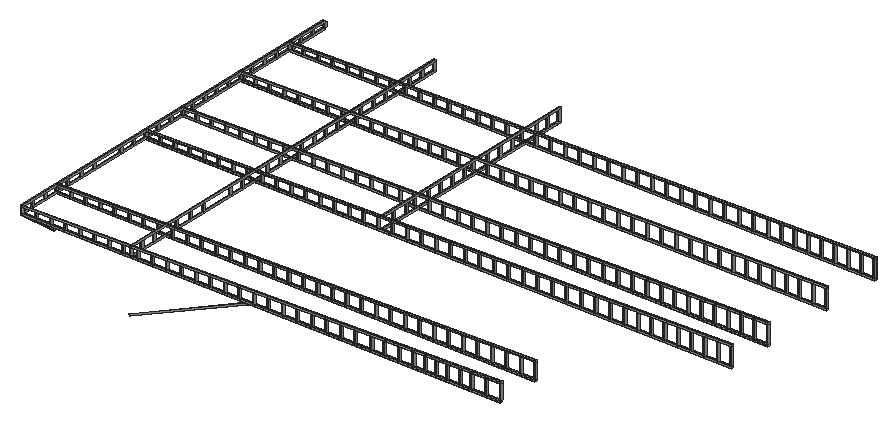
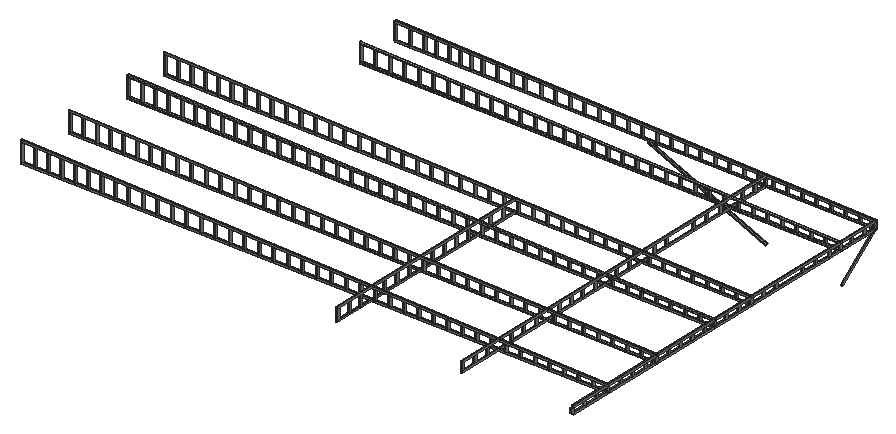
# SketchUp Ruby script. Lengths in millimetres.
U = 1.mm
M = Sketchup.active_model
def pt(a) = Geom::Point3d.new(a.map { |v| v * U })
def face(e, loops, mat)
  f = e.add_face(loops[0].map { |a| pt(a) })
  loops[1..].each { |l| e.add_face(l.map { |a| pt(a) }).erase! }
  f.material = f.back_material = mat if mat
  f
end
# faces: each face lists its corners as indices into pts; further lists are holes
def faces(e, pts, list, mat = nil) = list.each { |f| face(e, (f[0].is_a?(Array) ? f : [f]).map { |l| l.map { |i| pts[i] } }, mat) }
# xy, xz, yz: faces in a plane at the given z, y or x. An outline is a flat list of corners, or four numbers for a rectangle; further outlines are holes
def ring(l) = l.size == 4 ? [[l[0], l[1]], [l[2], l[1]], [l[2], l[3]], [l[0], l[3]]] : l.each_slice(2).to_a
def flat(e, list, mat, &to3) = list.each { |f| face(e, (f[0].is_a?(Array) ? f : [f]).map { |l| ring(l).map { |u, v| to3.(u, v) } }, mat) }
def xy(e, z, list, mat = nil) = flat(e, list, mat) { |x, y| [x, y, z] }
def xz(e, y, list, mat = nil) = flat(e, list, mat) { |x, z| [x, y, z] }
def yz(e, x, list, mat = nil) = flat(e, list, mat) { |y, z| [x, y, z] }
def lines(e, pts, list) = list.each { |a, b| e.add_line(pt(pts[a]), pt(pts[b])) }
# prism: a flat outline (further loops are holes) pulled along v
def prism(e, loops, v, mat = nil)
  f = face(e, loops, mat); d = Geom::Vector3d.new(v.map { |x| x * U })
  f.pushpull(f.normal.samedirection?(d) ? d.length : -d.length)
end
def box(e, o, s, mat = nil) = prism(e, [[o, [o[0] + s[0], o[1], o[2]], [o[0] + s[0], o[1] + s[1], o[2]], [o[0], o[1] + s[1], o[2]]]], [0, 0, s[2]], mat)
def at(x, y, z, deg = 0) = Geom::Transformation.translation(pt([x, y, z])) * Geom::Transformation.rotation(ORIGIN, Z_AXIS, deg.degrees)
def axes(o, x, y, z) = Geom::Transformation.new([*x, 0, *y, 0, *z, 0, *pt(o).to_a, 1])
def part(name) = M.definitions.add(name)
# library, detail: a bought-in or finely detailed component or shape, given as its bounding box
def library(name, o, s) = part(name).tap { |d| box(d.entities, o, s) }
def detail(e, o, s) = box(e.add_group.entities, o, s)
def put(e, d, t, mat = nil) = e.add_instance(d, t).tap { |i| i.material = mat if mat }
def group(e, t, mat = nil) = e.add_group.tap { |g| g.transformation = t; g.material = mat if mat }.entities
root = M.entities
M.materials.add("[Metal Rough]").color = [153, 157, 160]
c1 = part("Group\#22")
g1 = group(c1.entities,at(0,0,300))
prism(g1,[[[27087.5,80,600],[0,80,0],[0,80,80],[27087.5,80,680]]],[0,-80,0])
g2 = group(c1.entities,at(27087.5,0,0),"[Metal Rough]")
prism(g2,[[[-27087.5,80,0],[-27087.5,0,0],[-27087.5,0,80],[-27087.5,80,80]],[[-27087.5,76,4],[-27087.5,76,76],[-27087.5,4,76],[-27087.5,4,4]]],[27087.5,0,0])
c2 = part("Group\#63")
prism(c2.entities,[[[6104.2,85,80],[6104.2,85,435.2],[6078.7,85,434.6],[6024.2,85,433.4],[6024.2,85,80]]],[0,80,0],"[Metal Rough]")
prism(c2.entities,[[[7442.9,85,80],[7442.9,85,464.9],[7417.4,85,464.3],[7362.9,85,463.1],[7362.9,85,80]]],[0,80,0],"[Metal Rough]")
prism(c2.entities,[[[6773.6,85,80],[6773.6,85,450],[6748.1,85,449.5],[6693.6,85,448.3],[6693.6,85,80]]],[0,80,0],"[Metal Rough]")
prism(c2.entities,[[[8112.3,85,80],[8112.3,85,479.7],[8086.8,85,479.1],[8032.3,85,477.9],[8032.3,85,80]]],[0,80,0],"[Metal Rough]")
prism(c2.entities,[[[5434.8,85,80],[5434.8,85,420.4],[5409.4,85,419.8],[5354.8,85,418.6],[5354.8,85,80]]],[0,80,0],"[Metal Rough]")
prism(c2.entities,[[[4096.1,85,80],[4096.1,85,390.7],[4070.6,85,390.2],[4016.1,85,388.9],[4016.1,85,80]]],[0,80,0],"[Metal Rough]")
prism(c2.entities,[[[1418.7,165,80],[1338.7,165,80],[1338.7,165,329.6],[1393.2,165,330.9],[1418.7,165,331.4]]],[0,-80,0],"[Metal Rough]")
prism(c2.entities,[[[3426.8,165,80],[3346.8,165,80],[3346.8,165,374.1],[3401.3,165,375.3],[3426.8,165,375.9]]],[0,-80,0],"[Metal Rough]")
prism(c2.entities,[[[2757.4,165,80],[2677.4,165,80],[2677.4,165,359.3],[2731.9,165,360.5],[2757.4,165,361.1]]],[0,-80,0],"[Metal Rough]")
prism(c2.entities,[[[2088.1,165,80],[2008.1,165,80],[2008.1,165,344.5],[2062.6,165,345.7],[2088.1,165,346.2]]],[0,-80,0],"[Metal Rough]")
prism(c2.entities,[[[4765.5,85,80],[4765.5,85,405.5],[4740,85,405],[4685.5,85,403.8],[4685.5,85,80]]],[0,80,0],"[Metal Rough]")
prism(c2.entities,[[[80,85,80],[80,85,301.8],[0,85,300],[0,85,80]]],[0,80,0],"[Metal Rough]")
prism(c2.entities,[[[749.4,85,80],[749.4,85,316.6],[669.4,85,314.8],[669.4,85,80]]],[0,80,0],"[Metal Rough]")
prism(c2.entities,[[[12128.4,85,80],[12128.4,85,568.6],[12102.9,85,568.1],[12048.4,85,566.9],[12048.4,85,80]]],[0,80,0],"[Metal Rough]")
prism(c2.entities,[[[10120.3,165,80],[10040.3,165,80],[10040.3,165,522.4],[10094.9,165,523.6],[10120.3,165,524.2]]],[0,-80,0],"[Metal Rough]")
prism(c2.entities,[[[12797.8,85,80],[12797.8,85,583.5],[12772.3,85,582.9],[12717.8,85,581.7],[12717.8,85,80]]],[0,80,0],"[Metal Rough]")
prism(c2.entities,[[[24013.3,85,80],[24013.3,85,831.9],[23933.3,85,830.1],[23933.3,85,80]]],[0,80,0],"[Metal Rough]")
prism(c2.entities,[[[20160.7,165,80],[20080.7,165,80],[20080.7,165,744.8],[20135.2,165,746],[20160.7,165,746.6]]],[0,-80,0],"[Metal Rough]")
prism(c2.entities,[[[20830,165,80],[20750,165,80],[20750,165,759.6],[20804.6,165,760.8],[20830,165,761.4]]],[0,-80,0],"[Metal Rough]")
prism(c2.entities,[[[18152.6,165,80],[18072.6,165,80],[18072.6,165,700.3],[18127.1,165,701.5],[18152.6,165,702.1]]],[0,-80,0],"[Metal Rough]")
prism(c2.entities,[[[21499.4,165,80],[21419.4,165,80],[21419.4,165,774.4],[21473.9,165,775.6],[21499.4,165,776.2]]],[0,-80,0],"[Metal Rough]")
prism(c2.entities,[[[15475.2,165,80],[15395.2,165,80],[15395.2,165,641],[15449.7,165,642.2],[15475.2,165,642.8]]],[0,-80,0],"[Metal Rough]")
prism(c2.entities,[[[19491.3,165,80],[19411.3,165,80],[19411.3,165,730],[19465.8,165,731.2],[19491.3,165,731.7]]],[0,-80,0],"[Metal Rough]")
prism(c2.entities,[[[16813.9,165,80],[16733.9,165,80],[16733.9,165,670.7],[16788.4,165,671.9],[16813.9,165,672.4]]],[0,-80,0],"[Metal Rough]")
prism(c2.entities,[[[16144.5,165,80],[16064.5,165,80],[16064.5,165,655.8],[16119.1,165,657],[16144.5,165,657.6]]],[0,-80,0],"[Metal Rough]")
prism(c2.entities,[[[17483.3,165,80],[17403.3,165,80],[17403.3,165,685.5],[17457.8,165,686.7],[17483.3,165,687.3]]],[0,-80,0],"[Metal Rough]")
prism(c2.entities,[[[14805.8,165,80],[14725.8,165,80],[14725.8,165,626.2],[14780.3,165,627.4],[14805.8,165,627.9]]],[0,-80,0],"[Metal Rough]")
prism(c2.entities,[[[18822,165,80],[18742,165,80],[18742,165,715.1],[18796.5,165,716.3],[18822,165,716.9]]],[0,-80,0],"[Metal Rough]")
prism(c2.entities,[[[10789.7,165,80],[10709.7,165,80],[10709.7,165,537.2],[10764.2,165,538.4],[10789.7,165,539]]],[0,-80,0],"[Metal Rough]")
prism(c2.entities,[[[8781.6,165,80],[8701.6,165,80],[8701.6,165,492.7],[8756.1,165,493.9],[8781.6,165,494.5]]],[0,-80,0],"[Metal Rough]")
prism(c2.entities,[[[9451,165,80],[9371,165,80],[9371,165,507.6],[9425.5,165,508.8],[9451,165,509.3]]],[0,-80,0],"[Metal Rough]")
prism(c2.entities,[[[13467.1,165,80],[13387.1,165,80],[13387.1,165,596.5],[13441.6,165,597.7],[13467.1,165,598.3]]],[0,-80,0],"[Metal Rough]")
prism(c2.entities,[[[14136.5,165,80],[14056.5,165,80],[14056.5,165,611.3],[14111,165,612.6],[14136.5,165,613.1]]],[0,-80,0],"[Metal Rough]")
prism(c2.entities,[[[11459.1,165,80],[11379.1,165,80],[11379.1,165,552],[11433.6,165,553.2],[11459.1,165,553.8]]],[0,-80,0],"[Metal Rough]")
prism(c2.entities,[[[27087.5,85,80],[27087.5,85,900],[27007.5,85,897.8],[27007.5,85,80]]],[0,80,0],"[Metal Rough]")
prism(c2.entities,[[[26472.7,165,80],[26392.7,165,80],[26392.7,165,884.6],[26472.7,165,886.4]]],[0,-80,0],"[Metal Rough]")
prism(c2.entities,[[[25857.8,165,80],[25777.8,165,80],[25777.8,165,871],[25857.8,165,872.8]]],[0,-80,0],"[Metal Rough]")
prism(c2.entities,[[[22168.7,165,80],[22088.7,165,80],[22088.8,165,789.3],[22168.8,165,791]]],[0,-80,0],"[Metal Rough]")
prism(c2.entities,[[[25243,165,80],[25163,165,80],[25163,165,857.4],[25243,165,859.1]]],[0,-80,0],"[Metal Rough]")
prism(c2.entities,[[[24628.1,165,80],[24548.1,165,80],[24548.1,165,843.7],[24628.1,165,845.5]]],[0,-80,0],"[Metal Rough]")
prism(c2.entities,[[[22783.6,85,80],[22783.6,85,804.7],[22703.6,85,802.9],[22703.6,85,80]]],[0,80,0],"[Metal Rough]")
prism(c2.entities,[[[23398.4,165,80],[23318.4,165,80],[23318.4,165,816.5],[23398.4,165,818.3]]],[0,-80,0],"[Metal Rough]")
p = [[21499.4,85,776.2],[21553.9,85,777.4]]
lines(c2.entities,p,[[0,1]])
put(c2.entities,c1,at(0,85,0),"[Metal Rough]")
c3 = part("Group\#7")
prism(c3.entities,[[[0,0,4955],[0,80,4955],[80,80,4955],[80,0,4955]],[[76,76,4955],[4,76,4955],[4,4,4955],[76,4,4955]]],[0,0,22132.5])
c4 = part("Group\#57")
box(c4.entities,[0,0,0],[80,80,820])
c5 = part("Group\#49")
box(c5.entities,[0,0,0],[80,17546,80])
c6 = part("Group\#48")
box(c6.entities,[0,0,0],[80,17546,80])
g3 = group(root,at(12218.2,2438,2926.7),"[Metal Rough]")
prism(g3,[[[0,0,0],[-31.9,0,73.3],[-5440,0,-2281.5],[-5408.1,0,-2354.9]]],[0,80,0])
g4 = group(root,at(1756.3,4303.6,1540),"[Metal Rough]")
prism(g4,[[[0,51.9,-40.7],[0,101.3,22.2],[66.2,101.3,22.2],[66.2,51.9,-40.7]]],[0,-1914.4,1501.1])
put(root,c2,at(1756.3,14961,3000))
put(root,c2,at(1756.3,17759,3000))
put(root,c2,at(1756.3,11603,3000))
g5 = group(root,at(1756.3,9498.8,3000))
prism(g5,[[[6104.2,85,80],[6104.2,85,435.2],[6078.7,85,434.6],[6024.2,85,433.4],[6024.2,85,80]]],[0,80,0],"[Metal Rough]")
prism(g5,[[[7442.9,85,80],[7442.9,85,464.9],[7417.4,85,464.3],[7362.9,85,463.1],[7362.9,85,80]]],[0,80,0],"[Metal Rough]")
prism(g5,[[[6773.6,85,80],[6773.6,85,450],[6748.1,85,449.5],[6693.6,85,448.3],[6693.6,85,80]]],[0,80,0],"[Metal Rough]")
prism(g5,[[[8112.3,85,80],[8112.3,85,479.7],[8086.8,85,479.1],[8032.3,85,477.9],[8032.3,85,80]]],[0,80,0],"[Metal Rough]")
prism(g5,[[[5434.8,85,80],[5434.8,85,420.4],[5409.4,85,419.8],[5354.8,85,418.6],[5354.8,85,80]]],[0,80,0],"[Metal Rough]")
prism(g5,[[[4096.1,85,80],[4096.1,85,390.7],[4070.6,85,390.2],[4016.1,85,388.9],[4016.1,85,80]]],[0,80,0],"[Metal Rough]")
prism(g5,[[[1418.7,165,80],[1338.7,165,80],[1338.7,165,329.6],[1393.2,165,330.9],[1418.7,165,331.4]]],[0,-80,0],"[Metal Rough]")
prism(g5,[[[3426.8,165,80],[3346.8,165,80],[3346.8,165,374.1],[3401.3,165,375.3],[3426.8,165,375.9]]],[0,-80,0],"[Metal Rough]")
prism(g5,[[[2757.4,165,80],[2677.4,165,80],[2677.4,165,359.3],[2731.9,165,360.5],[2757.4,165,361.1]]],[0,-80,0],"[Metal Rough]")
prism(g5,[[[2088.1,165,80],[2008.1,165,80],[2008.1,165,344.5],[2062.6,165,345.7],[2088.1,165,346.2]]],[0,-80,0],"[Metal Rough]")
prism(g5,[[[4765.5,85,80],[4765.5,85,405.5],[4740,85,405],[4685.5,85,403.8],[4685.5,85,80]]],[0,80,0],"[Metal Rough]")
prism(g5,[[[80,85,80],[80,85,301.8],[0,85,300],[0,85,80]]],[0,80,0],"[Metal Rough]")
prism(g5,[[[749.4,85,80],[749.4,85,316.6],[669.4,85,314.8],[669.4,85,80]]],[0,80,0],"[Metal Rough]")
prism(g5,[[[12128.4,85,80],[12128.4,85,568.6],[12102.9,85,568.1],[12048.4,85,566.9],[12048.4,85,80]]],[0,80,0],"[Metal Rough]")
prism(g5,[[[10120.3,165,80],[10040.3,165,80],[10040.3,165,522.4],[10094.9,165,523.6],[10120.3,165,524.2]]],[0,-80,0],"[Metal Rough]")
prism(g5,[[[12797.8,85,80],[12797.8,85,583.5],[12772.3,85,582.9],[12717.8,85,581.7],[12717.8,85,80]]],[0,80,0],"[Metal Rough]")
prism(g5,[[[24013.3,85,80],[24013.3,85,831.9],[23933.3,85,830.1],[23933.3,85,80]]],[0,80,0],"[Metal Rough]")
prism(g5,[[[20160.7,165,80],[20080.7,165,80],[20080.7,165,744.8],[20135.2,165,746],[20160.7,165,746.6]]],[0,-80,0],"[Metal Rough]")
prism(g5,[[[20830,165,80],[20750,165,80],[20750,165,759.6],[20804.6,165,760.8],[20830,165,761.4]]],[0,-80,0],"[Metal Rough]")
prism(g5,[[[18152.6,165,80],[18072.6,165,80],[18072.6,165,700.3],[18127.1,165,701.5],[18152.6,165,702.1]]],[0,-80,0],"[Metal Rough]")
prism(g5,[[[21499.4,165,80],[21419.4,165,80],[21419.4,165,774.4],[21473.9,165,775.6],[21499.4,165,776.2]]],[0,-80,0],"[Metal Rough]")
prism(g5,[[[15475.2,165,80],[15395.2,165,80],[15395.2,165,641],[15449.7,165,642.2],[15475.2,165,642.8]]],[0,-80,0],"[Metal Rough]")
prism(g5,[[[19491.3,165,80],[19411.3,165,80],[19411.3,165,730],[19465.8,165,731.2],[19491.3,165,731.7]]],[0,-80,0],"[Metal Rough]")
prism(g5,[[[16813.9,165,80],[16733.9,165,80],[16733.9,165,670.7],[16788.4,165,671.9],[16813.9,165,672.4]]],[0,-80,0],"[Metal Rough]")
prism(g5,[[[16144.5,165,80],[16064.5,165,80],[16064.5,165,655.8],[16119.1,165,657],[16144.5,165,657.6]]],[0,-80,0],"[Metal Rough]")
prism(g5,[[[17483.3,165,80],[17403.3,165,80],[17403.3,165,685.5],[17457.8,165,686.7],[17483.3,165,687.3]]],[0,-80,0],"[Metal Rough]")
prism(g5,[[[14805.8,165,80],[14725.8,165,80],[14725.8,165,626.2],[14780.3,165,627.4],[14805.8,165,627.9]]],[0,-80,0],"[Metal Rough]")
prism(g5,[[[18822,165,80],[18742,165,80],[18742,165,715.1],[18796.5,165,716.3],[18822,165,716.9]]],[0,-80,0],"[Metal Rough]")
prism(g5,[[[10789.7,165,80],[10709.7,165,80],[10709.7,165,537.2],[10764.2,165,538.4],[10789.7,165,539]]],[0,-80,0],"[Metal Rough]")
prism(g5,[[[8781.6,165,80],[8701.6,165,80],[8701.6,165,492.7],[8756.1,165,493.9],[8781.6,165,494.5]]],[0,-80,0],"[Metal Rough]")
prism(g5,[[[9451,165,80],[9371,165,80],[9371,165,507.6],[9425.5,165,508.8],[9451,165,509.3]]],[0,-80,0],"[Metal Rough]")
prism(g5,[[[13467.1,165,80],[13387.1,165,80],[13387.1,165,596.5],[13441.6,165,597.7],[13467.1,165,598.3]]],[0,-80,0],"[Metal Rough]")
prism(g5,[[[14136.5,165,80],[14056.5,165,80],[14056.5,165,611.3],[14111,165,612.6],[14136.5,165,613.1]]],[0,-80,0],"[Metal Rough]")
prism(g5,[[[11459.1,165,80],[11379.1,165,80],[11379.1,165,552],[11433.6,165,553.2],[11459.1,165,553.8]]],[0,-80,0],"[Metal Rough]")
prism(g5,[[[27087.5,85,80],[27087.5,85,900],[27007.5,85,897.8],[27007.5,85,80]]],[0,80,0],"[Metal Rough]")
prism(g5,[[[26472.7,165,80],[26392.7,165,80],[26392.7,165,884.6],[26472.7,165,886.4]]],[0,-80,0],"[Metal Rough]")
prism(g5,[[[25857.8,165,80],[25777.8,165,80],[25777.8,165,871],[25857.8,165,872.8]]],[0,-80,0],"[Metal Rough]")
prism(g5,[[[22168.7,165,80],[22088.7,165,80],[22088.8,165,789.3],[22168.8,165,791]]],[0,-80,0],"[Metal Rough]")
prism(g5,[[[25243,165,80],[25163,165,80],[25163,165,857.4],[25243,165,859.1]]],[0,-80,0],"[Metal Rough]")
prism(g5,[[[24628.1,165,80],[24548.1,165,80],[24548.1,165,843.7],[24628.1,165,845.5]]],[0,-80,0],"[Metal Rough]")
prism(g5,[[[22783.6,85,80],[22783.6,85,804.7],[22703.6,85,802.9],[22703.6,85,80]]],[0,80,0],"[Metal Rough]")
prism(g5,[[[23398.4,165,80],[23318.4,165,80],[23318.4,165,816.5],[23398.4,165,818.3]]],[0,-80,0],"[Metal Rough]")
p = [[21499.4,85,776.2],[21553.9,85,777.4]]
lines(g5,p,[[0,1]])
put(g5,c1,at(0,85,0),"[Metal Rough]")
g6 = group(root,at(1756.3,2353,3000))
prism(g6,[[[6104.2,85,80],[6104.2,85,435.2],[6078.7,85,434.6],[6024.2,85,433.4],[6024.2,85,80]]],[0,80,0],"[Metal Rough]")
prism(g6,[[[7442.9,85,80],[7442.9,85,464.9],[7417.4,85,464.3],[7362.9,85,463.1],[7362.9,85,80]]],[0,80,0],"[Metal Rough]")
prism(g6,[[[6773.6,85,80],[6773.6,85,450],[6748.1,85,449.5],[6693.6,85,448.3],[6693.6,85,80]]],[0,80,0],"[Metal Rough]")
prism(g6,[[[8112.3,85,80],[8112.3,85,479.7],[8086.8,85,479.1],[8032.3,85,477.9],[8032.3,85,80]]],[0,80,0],"[Metal Rough]")
prism(g6,[[[5434.8,85,80],[5434.8,85,420.4],[5409.4,85,419.8],[5354.8,85,418.6],[5354.8,85,80]]],[0,80,0],"[Metal Rough]")
prism(g6,[[[4096.1,85,80],[4096.1,85,390.7],[4070.6,85,390.2],[4016.1,85,388.9],[4016.1,85,80]]],[0,80,0],"[Metal Rough]")
prism(g6,[[[1418.7,165,80],[1338.7,165,80],[1338.7,165,329.6],[1393.2,165,330.9],[1418.7,165,331.4]]],[0,-80,0],"[Metal Rough]")
prism(g6,[[[3426.8,165,80],[3346.8,165,80],[3346.8,165,374.1],[3401.3,165,375.3],[3426.8,165,375.9]]],[0,-80,0],"[Metal Rough]")
prism(g6,[[[2757.4,165,80],[2677.4,165,80],[2677.4,165,359.3],[2731.9,165,360.5],[2757.4,165,361.1]]],[0,-80,0],"[Metal Rough]")
prism(g6,[[[2088.1,165,80],[2008.1,165,80],[2008.1,165,344.5],[2062.6,165,345.7],[2088.1,165,346.2]]],[0,-80,0],"[Metal Rough]")
prism(g6,[[[4765.5,85,80],[4765.5,85,405.5],[4740,85,405],[4685.5,85,403.8],[4685.5,85,80]]],[0,80,0],"[Metal Rough]")
prism(g6,[[[80,85,80],[80,85,301.8],[0,85,300],[0,85,80]]],[0,80,0],"[Metal Rough]")
prism(g6,[[[749.4,85,80],[749.4,85,316.6],[669.4,85,314.8],[669.4,85,80]]],[0,80,0],"[Metal Rough]")
prism(g6,[[[12128.4,85,80],[12128.4,85,568.6],[12102.9,85,568.1],[12048.4,85,566.9],[12048.4,85,80]]],[0,80,0],"[Metal Rough]")
prism(g6,[[[10120.3,165,80],[10040.3,165,80],[10040.3,165,522.4],[10094.9,165,523.6],[10120.3,165,524.2]]],[0,-80,0],"[Metal Rough]")
prism(g6,[[[12797.8,85,80],[12797.8,85,583.5],[12772.3,85,582.9],[12717.8,85,581.7],[12717.8,85,80]]],[0,80,0],"[Metal Rough]")
prism(g6,[[[20294.7,165,80],[20214.7,165,80],[20214.7,165,744.8],[20269.2,165,746],[20294.7,165,746.6]]],[0,-80,0],"[Metal Rough]")
prism(g6,[[[20830,165,80],[20750,165,80],[20750,165,759.6],[20804.6,165,760.8],[20830,165,761.4]]],[0,-80,0],"[Metal Rough]")
prism(g6,[[[18152.6,165,80],[18072.6,165,80],[18072.6,165,700.3],[18127.1,165,701.5],[18152.6,165,702.1]]],[0,-80,0],"[Metal Rough]")
prism(g6,[[[21499.4,165,80],[21419.4,165,80],[21419.4,165,774.4],[21473.9,165,775.6],[21499.4,165,776.2]]],[0,-80,0],"[Metal Rough]")
prism(g6,[[[15475.2,165,80],[15395.2,165,80],[15395.2,165,641],[15449.7,165,642.2],[15475.2,165,642.8]]],[0,-80,0],"[Metal Rough]")
prism(g6,[[[19195.1,165,80],[19115.1,165,80],[19115.1,165,730],[19169.6,165,731.2],[19195.1,165,731.7]]],[0,-80,0],"[Metal Rough]")
prism(g6,[[[16813.9,165,80],[16733.9,165,80],[16733.9,165,670.7],[16788.4,165,671.9],[16813.9,165,672.4]]],[0,-80,0],"[Metal Rough]")
prism(g6,[[[16217.6,165,80],[16137.6,165,80],[16137.6,165,655.8],[16192.1,165,657],[16217.6,165,657.6]]],[0,-80,0],"[Metal Rough]")
prism(g6,[[[17483.3,165,80],[17403.3,165,80],[17403.3,165,685.5],[17457.8,165,686.7],[17483.3,165,687.3]]],[0,-80,0],"[Metal Rough]")
prism(g6,[[[14805.8,165,80],[14725.8,165,80],[14725.8,165,626.2],[14780.3,165,627.4],[14805.8,165,627.9]]],[0,-80,0],"[Metal Rough]")
prism(g6,[[[18701,165,80],[18621,165,80],[18621,165,715.1],[18675.5,165,716.3],[18701,165,716.9]]],[0,-80,0],"[Metal Rough]")
prism(g6,[[[10789.7,165,80],[10709.7,165,80],[10709.7,165,537.2],[10764.2,165,538.4],[10789.7,165,539]]],[0,-80,0],"[Metal Rough]")
prism(g6,[[[8781.6,165,80],[8701.6,165,80],[8701.6,165,492.7],[8756.1,165,493.9],[8781.6,165,494.5]]],[0,-80,0],"[Metal Rough]")
prism(g6,[[[9451,165,80],[9371,165,80],[9371,165,507.6],[9425.5,165,508.8],[9451,165,509.3]]],[0,-80,0],"[Metal Rough]")
prism(g6,[[[13467.1,165,80],[13387.1,165,80],[13387.1,165,596.5],[13441.6,165,597.7],[13467.1,165,598.3]]],[0,-80,0],"[Metal Rough]")
prism(g6,[[[14136.5,165,80],[14056.5,165,80],[14056.5,165,611.3],[14111,165,612.6],[14136.5,165,613.1]]],[0,-80,0],"[Metal Rough]")
prism(g6,[[[11459.1,165,80],[11379.1,165,80],[11379.1,165,552],[11433.6,165,553.2],[11459.1,165,553.8]]],[0,-80,0],"[Metal Rough]")
prism(g6,[[[22172.5,165,80],[22092.5,165,80],[22092.5,165,788.5],[22172.5,165,790.2]]],[0,-80,0],"[Metal Rough]")
prism(g6,[[[19705.1,165,80],[19625.1,165,80],[19625.1,165,730],[19679.6,165,731.2],[19705.1,165,731.7]]],[0,-80,0],"[Metal Rough]")
p = [[21499.4,85,776.2],[21553.9,85,777.4]]
lines(g6,p,[[0,1]])
g7 = group(g6,at(0,85,0),"[Metal Rough]")
g8 = group(g7,at(0,0,300))
prism(g8,[[[0,80,80],[22132.5,80,570.3],[22172.5,80,570.3],[22172.5,80,490.2],[22132.5,80,490.2],[0,80,0]]],[0,-80,0])
put(g7,c3,axes([27087.5,0,0],[0,0,1],[0,1,0],[-1,0,0]),"[Metal Rough]")
g9 = group(root,at(1756.3,4353,3000))
prism(g9,[[[6104.2,85,80],[6104.2,85,435.2],[6078.7,85,434.6],[6024.2,85,433.4],[6024.2,85,80]]],[0,80,0],"[Metal Rough]")
prism(g9,[[[7442.9,85,80],[7442.9,85,464.9],[7417.4,85,464.3],[7362.9,85,463.1],[7362.9,85,80]]],[0,80,0],"[Metal Rough]")
prism(g9,[[[6773.6,85,80],[6773.6,85,450],[6748.1,85,449.5],[6693.6,85,448.3],[6693.6,85,80]]],[0,80,0],"[Metal Rough]")
prism(g9,[[[8112.3,85,80],[8112.3,85,479.7],[8086.8,85,479.1],[8032.3,85,477.9],[8032.3,85,80]]],[0,80,0],"[Metal Rough]")
prism(g9,[[[5434.8,85,80],[5434.8,85,420.4],[5409.4,85,419.8],[5354.8,85,418.6],[5354.8,85,80]]],[0,80,0],"[Metal Rough]")
prism(g9,[[[4096.1,85,80],[4096.1,85,390.7],[4070.6,85,390.2],[4016.1,85,388.9],[4016.1,85,80]]],[0,80,0],"[Metal Rough]")
prism(g9,[[[1418.7,165,80],[1338.7,165,80],[1338.7,165,329.6],[1393.2,165,330.9],[1418.7,165,331.4]]],[0,-80,0],"[Metal Rough]")
prism(g9,[[[3426.8,165,80],[3346.8,165,80],[3346.8,165,374.1],[3401.3,165,375.3],[3426.8,165,375.9]]],[0,-80,0],"[Metal Rough]")
prism(g9,[[[2757.4,165,80],[2677.4,165,80],[2677.4,165,359.3],[2731.9,165,360.5],[2757.4,165,361.1]]],[0,-80,0],"[Metal Rough]")
prism(g9,[[[2088.1,165,80],[2008.1,165,80],[2008.1,165,344.5],[2062.6,165,345.7],[2088.1,165,346.2]]],[0,-80,0],"[Metal Rough]")
prism(g9,[[[4765.5,85,80],[4765.5,85,405.5],[4740,85,405],[4685.5,85,403.8],[4685.5,85,80]]],[0,80,0],"[Metal Rough]")
prism(g9,[[[80,85,80],[80,85,301.8],[0,85,300],[0,85,80]]],[0,80,0],"[Metal Rough]")
prism(g9,[[[749.4,85,80],[749.4,85,316.6],[669.4,85,314.8],[669.4,85,80]]],[0,80,0],"[Metal Rough]")
prism(g9,[[[12128.4,85,80],[12128.4,85,568.6],[12102.9,85,568.1],[12048.4,85,566.9],[12048.4,85,80]]],[0,80,0],"[Metal Rough]")
prism(g9,[[[10120.3,165,80],[10040.3,165,80],[10040.3,165,522.4],[10094.9,165,523.6],[10120.3,165,524.2]]],[0,-80,0],"[Metal Rough]")
prism(g9,[[[12797.8,85,80],[12797.8,85,583.5],[12772.3,85,582.9],[12717.8,85,581.7],[12717.8,85,80]]],[0,80,0],"[Metal Rough]")
prism(g9,[[[20160.7,165,80],[20080.7,165,80],[20080.7,165,744.8],[20135.2,165,746],[20160.7,165,746.6]]],[0,-80,0],"[Metal Rough]")
prism(g9,[[[20830,165,80],[20750,165,80],[20750,165,759.6],[20804.6,165,760.8],[20830,165,761.4]]],[0,-80,0],"[Metal Rough]")
prism(g9,[[[18152.6,165,80],[18072.6,165,80],[18072.6,165,700.3],[18127.1,165,701.5],[18152.6,165,702.1]]],[0,-80,0],"[Metal Rough]")
prism(g9,[[[21499.4,165,80],[21419.4,165,80],[21419.4,165,774.4],[21473.9,165,775.6],[21499.4,165,776.2]]],[0,-80,0],"[Metal Rough]")
prism(g9,[[[15475.2,165,80],[15395.2,165,80],[15395.2,165,641],[15449.7,165,642.2],[15475.2,165,642.8]]],[0,-80,0],"[Metal Rough]")
prism(g9,[[[19491.3,165,80],[19411.3,165,80],[19411.3,165,730],[19465.8,165,731.2],[19491.3,165,731.7]]],[0,-80,0],"[Metal Rough]")
prism(g9,[[[16813.9,165,80],[16733.9,165,80],[16733.9,165,670.7],[16788.4,165,671.9],[16813.9,165,672.4]]],[0,-80,0],"[Metal Rough]")
prism(g9,[[[16144.5,165,80],[16064.5,165,80],[16064.5,165,655.8],[16119.1,165,657],[16144.5,165,657.6]]],[0,-80,0],"[Metal Rough]")
prism(g9,[[[17483.3,165,80],[17403.3,165,80],[17403.3,165,685.5],[17457.8,165,686.7],[17483.3,165,687.3]]],[0,-80,0],"[Metal Rough]")
prism(g9,[[[14805.8,165,80],[14725.8,165,80],[14725.8,165,626.2],[14780.3,165,627.4],[14805.8,165,627.9]]],[0,-80,0],"[Metal Rough]")
prism(g9,[[[18822,165,80],[18742,165,80],[18742,165,715.1],[18796.5,165,716.3],[18822,165,716.9]]],[0,-80,0],"[Metal Rough]")
prism(g9,[[[10789.7,165,80],[10709.7,165,80],[10709.7,165,537.2],[10764.2,165,538.4],[10789.7,165,539]]],[0,-80,0],"[Metal Rough]")
prism(g9,[[[8781.6,165,80],[8701.6,165,80],[8701.6,165,492.7],[8756.1,165,493.9],[8781.6,165,494.5]]],[0,-80,0],"[Metal Rough]")
prism(g9,[[[9451,165,80],[9371,165,80],[9371,165,507.6],[9425.5,165,508.8],[9451,165,509.3]]],[0,-80,0],"[Metal Rough]")
prism(g9,[[[13467.1,165,80],[13387.1,165,80],[13387.1,165,596.5],[13441.6,165,597.7],[13467.1,165,598.3]]],[0,-80,0],"[Metal Rough]")
prism(g9,[[[14136.5,165,80],[14056.5,165,80],[14056.5,165,611.3],[14111,165,612.6],[14136.5,165,613.1]]],[0,-80,0],"[Metal Rough]")
prism(g9,[[[11459.1,165,80],[11379.1,165,80],[11379.1,165,552],[11433.6,165,553.2],[11459.1,165,553.8]]],[0,-80,0],"[Metal Rough]")
prism(g9,[[[22172.5,165,80],[22092.5,165,80],[22092.5,165,788.5],[22172.5,165,790.2]]],[0,-80,0],"[Metal Rough]")
p = [[21499.4,85,776.2],[21553.9,85,777.4]]
lines(g9,p,[[0,1]])
g10 = group(g9,at(0,85,0),"[Metal Rough]")
g11 = group(g10,at(0,0,300))
prism(g11,[[[0,80,80],[22132.5,80,570.3],[22172.5,80,570.3],[22172.5,80,490.2],[22132.5,80,490.2],[0,80,0]]],[0,-80,0])
put(g10,c3,axes([27087.5,0,0],[0,0,1],[0,1,0],[-1,0,0]),"[Metal Rough]")
g12 = group(root,at(1756.3,2438,3000))
g13 = group(g12,at(0,0,0),"[Metal Rough]")
box(g13,[0,0,0],[80,17434.8,80])
g14 = group(g12,at(0,0,301.8),"[Metal Rough]")
box(g14,[0,0,0],[80,17434.8,80])
g15 = group(g12,at(0,1326.8,80),"[Metal Rough]")
box(g15,[0,0,0],[80,80,221.8])
put(g12,c4,axes([0,619.8,80],[1,0,0],[0,1,0],[0,0,0.27046]),"[Metal Rough]")
put(g12,c4,axes([0,2630.8,80],[1,0,0],[0,1,0],[0,0,0.27046]),"[Metal Rough]")
put(g12,c4,axes([0,3409.8,80],[1,0,0],[0,1,0],[0,0,0.27046]),"[Metal Rough]")
put(g12,c4,axes([0,4163.8,80],[1,0,0],[0,1,0],[0,0,0.27046]),"[Metal Rough]")
put(g12,c4,axes([0,5701.8,80],[1,0,0],[0,1,0],[0,0,0.27046]),"[Metal Rough]")
put(g12,c4,axes([0,6439.8,80],[1,0,0],[0,1,0],[0,0,0.27046]),"[Metal Rough]")
put(g12,c4,axes([0,8583.8,80],[1,0,0],[0,1,0],[0,0,0.27046]),"[Metal Rough]")
put(g12,c4,axes([0,7834.8,80],[1,0,0],[0,1,0],[0,0,0.27046]),"[Metal Rough]")
put(g12,c4,axes([0,9830.8,80],[1,0,0],[0,1,0],[0,0,0.27046]),"[Metal Rough]")
put(g12,c4,axes([0,10547.8,80],[1,0,0],[0,1,0],[0,0,0.27046]),"[Metal Rough]")
put(g12,c4,axes([0,11219.8,80],[1,0,0],[0,1,0],[0,0,0.27046]),"[Metal Rough]")
put(g12,c4,axes([0,11903.8,80],[1,0,0],[0,1,0],[0,0,0.27046]),"[Metal Rough]")
put(g12,c4,axes([0,13240.8,80],[1,0,0],[0,1,0],[0,0,0.27046]),"[Metal Rough]")
put(g12,c4,axes([0,13957.8,80],[1,0,0],[0,1,0],[0,0,0.27046]),"[Metal Rough]")
put(g12,c4,axes([0,14664.8,80],[1,0,0],[0,1,0],[0,0,0.27046]),"[Metal Rough]")
put(g12,c4,axes([0,16044.8,80],[1,0,0],[0,1,0],[0,0,0.27046]),"[Metal Rough]")
put(g12,c4,axes([0,16762.8,80],[1,0,0],[0,1,0],[0,0,0.27046]),"[Metal Rough]")
put(g12,c4,axes([0,17466,80],[1,0,0],[0,1,0],[0,0,0.27046]),"[Metal Rough]")
g16 = group(root,at(12633.6,2438,3000))
g17 = group(g16,at(0,0,0),"[Metal Rough]")
box(g17,[0,7225.8,0],[80,10209,80])
g18 = group(g16,at(0,0,542.7),"[Metal Rough]")
box(g18,[0,7225.8,0],[80,10209,80])
put(g16,c4,axes([0,8583.8,80],[1,0,0],[0,1,0],[0,0,0.56428]),"[Metal Rough]")
put(g16,c4,axes([0,7834.8,80],[1,0,0],[0,1,0],[0,0,0.56428]),"[Metal Rough]")
put(g16,c4,axes([0,9830.8,80],[1,0,0],[0,1,0],[0,0,0.56428]),"[Metal Rough]")
put(g16,c4,axes([0,10547.8,80],[1,0,0],[0,1,0],[0,0,0.56428]),"[Metal Rough]")
put(g16,c4,axes([0,11219.8,80],[1,0,0],[0,1,0],[0,0,0.56428]),"[Metal Rough]")
put(g16,c4,axes([0,11903.8,80],[1,0,0],[0,1,0],[0,0,0.56428]),"[Metal Rough]")
put(g16,c4,axes([0,13240.8,80],[1,0,0],[0,1,0],[0,0,0.56428]),"[Metal Rough]")
put(g16,c4,axes([0,13957.8,80],[1,0,0],[0,1,0],[0,0,0.56428]),"[Metal Rough]")
put(g16,c4,axes([0,14664.8,80],[1,0,0],[0,1,0],[0,0,0.56428]),"[Metal Rough]")
put(g16,c4,axes([0,16044.8,80],[1,0,0],[0,1,0],[0,0,0.56428]),"[Metal Rough]")
put(g16,c4,axes([0,16695.8,80],[1,0,0],[0,1,0],[0,0,0.56428]),"[Metal Rough]")
put(g16,c4,axes([0,17354.8,80],[1,0,0],[0,1,0],[0,0,0.56428]),"[Metal Rough]")
g19 = group(root,at(6789.8,2438,3000))
put(g19,c5,at(0,0,0),"[Metal Rough]")
put(g19,c6,at(0,0,411.5),"[Metal Rough]")
put(g19,c4,axes([0,1326.8,80],[1,0,0],[0,1,0],[0,0,0.40427]),"[Metal Rough]")
put(g19,c4,axes([0,619.8,80],[1,0,0],[0,1,0],[0,0,0.40427]),"[Metal Rough]")
put(g19,c4,axes([0,2630.8,80],[1,0,0],[0,1,0],[0,0,0.40427]),"[Metal Rough]")
put(g19,c4,axes([0,3409.8,80],[1,0,0],[0,1,0],[0,0,0.40427]),"[Metal Rough]")
put(g19,c4,axes([0,4163.8,80],[1,0,0],[0,1,0],[0,0,0.40427]),"[Metal Rough]")
put(g19,c4,axes([0,5701.8,80],[1,0,0],[0,1,0],[0,0,0.40427]),"[Metal Rough]")
put(g19,c4,axes([0,6439.8,80],[1,0,0],[0,1,0],[0,0,0.40427]),"[Metal Rough]")
put(g19,c4,axes([0,8583.8,80],[1,0,0],[0,1,0],[0,0,0.40427]),"[Metal Rough]")
put(g19,c4,axes([0,7834.8,80],[1,0,0],[0,1,0],[0,0,0.40427]),"[Metal Rough]")
put(g19,c4,axes([0,9830.8,80],[1,0,0],[0,1,0],[0,0,0.40427]),"[Metal Rough]")
put(g19,c4,axes([0,10547.8,80],[1,0,0],[0,1,0],[0,0,0.40427]),"[Metal Rough]")
put(g19,c4,axes([0,11219.8,80],[1,0,0],[0,1,0],[0,0,0.40427]),"[Metal Rough]")
put(g19,c4,axes([0,11903.8,80],[1,0,0],[0,1,0],[0,0,0.40427]),"[Metal Rough]")
put(g19,c4,axes([0,13240.8,80],[1,0,0],[0,1,0],[0,0,0.40427]),"[Metal Rough]")
put(g19,c4,axes([0,13957.8,80],[1,0,0],[0,1,0],[0,0,0.40427]),"[Metal Rough]")
put(g19,c4,axes([0,14664.8,80],[1,0,0],[0,1,0],[0,0,0.40427]),"[Metal Rough]")
put(g19,c4,axes([0,16044.8,80],[1,0,0],[0,1,0],[0,0,0.40427]),"[Metal Rough]")
put(g19,c4,axes([0,16762.8,80],[1,0,0],[0,1,0],[0,0,0.40427]),"[Metal Rough]")
put(g19,c4,axes([0,17466,80],[1,0,0],[0,1,0],[0,0,0.40427]),"[Metal Rough]")
put(g19,c4,axes([0,0,80],[1,0,0],[0,1,0],[0,0,0.40427]),"[Metal Rough]")
g20 = group(root,at(6789.8,2438,3000),"[Metal Rough]")
box(g20,[0,0,0],[80,80,221.8])
